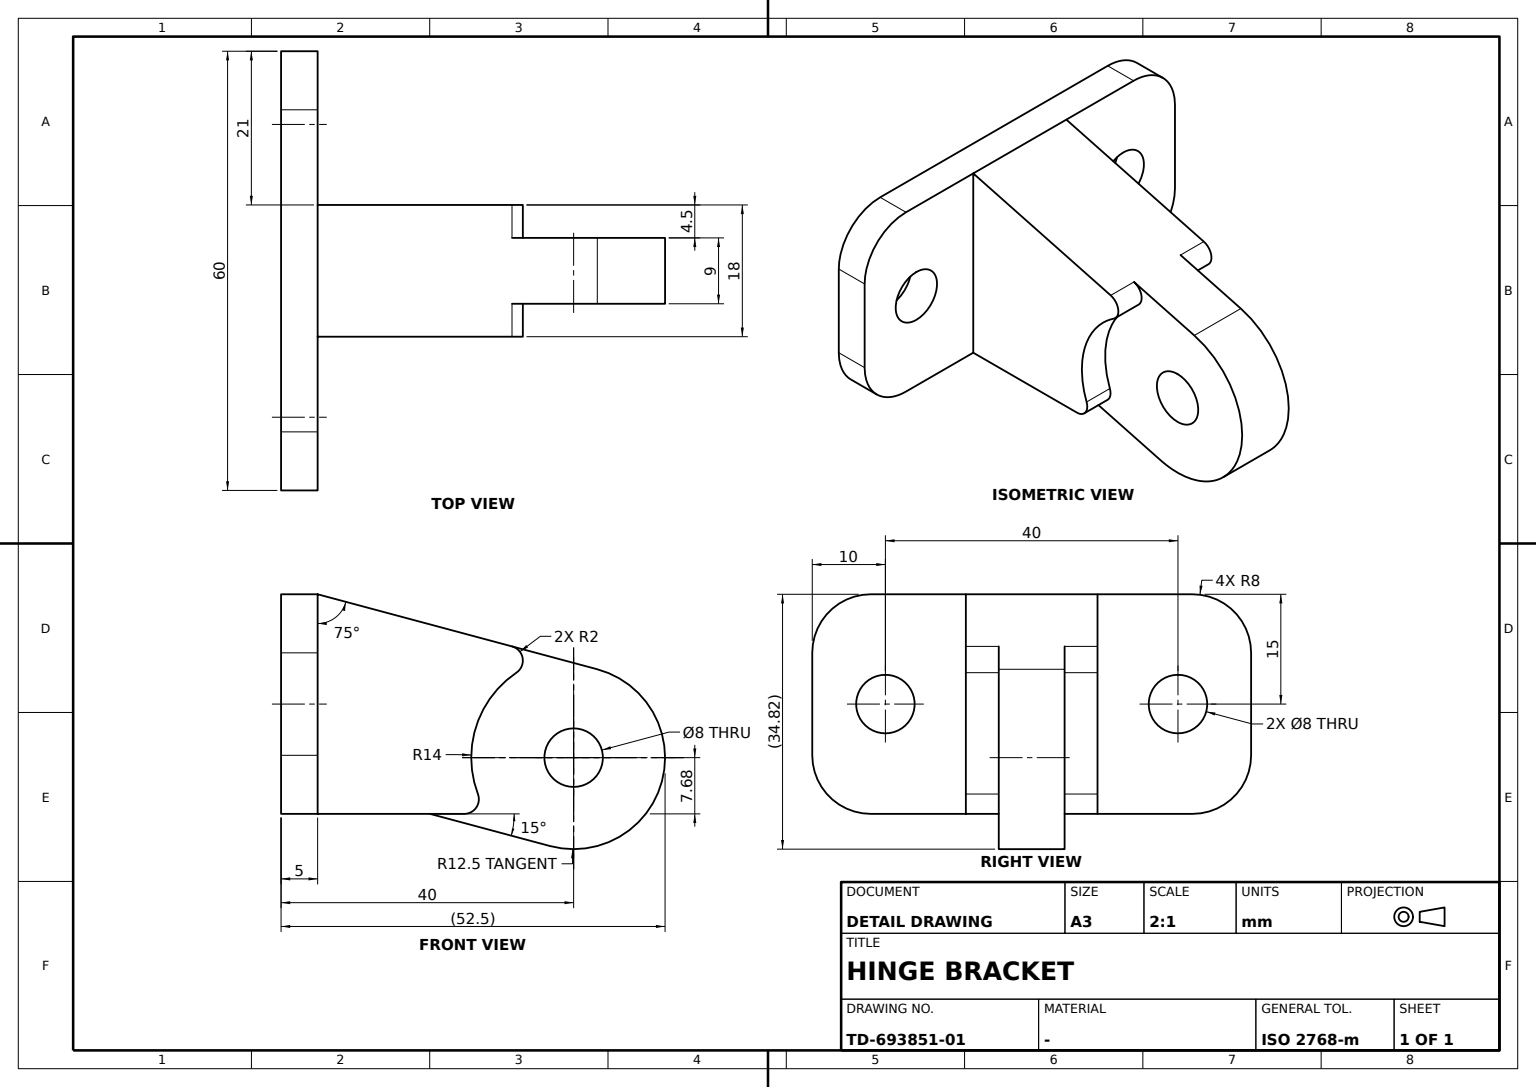
ISO-10303-21;
HEADER;
FILE_DESCRIPTION((''),'2;1');
FILE_NAME('','',(''),(''),'','','');
FILE_SCHEMA(('AUTOMOTIVE_DESIGN'));
ENDSEC;
DATA;
#1=APPLICATION_CONTEXT('');
#2=PRODUCT_CONTEXT('',#1,'mechanical');
#3=PRODUCT('','','',(#2));
#4=PRODUCT_DEFINITION_FORMATION('','',#3);
#5=PRODUCT_DEFINITION_CONTEXT('',#1,'design');
#6=PRODUCT_DEFINITION('','',#4,#5);
#7=PRODUCT_DEFINITION_SHAPE('','',#6);
#8=(LENGTH_UNIT()NAMED_UNIT(*)SI_UNIT(.MILLI.,.METRE.));
#9=(NAMED_UNIT(*)PLANE_ANGLE_UNIT()SI_UNIT($,.RADIAN.));
#10=(NAMED_UNIT(*)SI_UNIT($,.STERADIAN.)SOLID_ANGLE_UNIT());
#11=UNCERTAINTY_MEASURE_WITH_UNIT(LENGTH_MEASURE(0.005),#8,'distance_accuracy_value','');
#12=(GEOMETRIC_REPRESENTATION_CONTEXT(3)GLOBAL_UNCERTAINTY_ASSIGNED_CONTEXT((#11))GLOBAL_UNIT_ASSIGNED_CONTEXT((#8,#9,#10))REPRESENTATION_CONTEXT('',''));
#13=CARTESIAN_POINT('',(-4.5,-25.042453,-15.));
#14=VERTEX_POINT('',#13);
#15=CARTESIAN_POINT('',(-9.,-25.042453,-15.));
#16=VERTEX_POINT('',#15);
#17=CARTESIAN_POINT('',(9.,-25.042453,-15.));
#18=DIRECTION('',(-1.,0.,0.));
#19=VECTOR('',#18,1000.);
#20=LINE('',#17,#19);
#21=EDGE_CURVE('',#14,#16,#20,.T.);
#22=ORIENTED_EDGE('',*,*,#21,.F.);
#23=CARTESIAN_POINT('',(-4.5,-26.912146,-12.289897));
#24=VERTEX_POINT('',#23);
#25=CARTESIAN_POINT('',(-4.5,-25.042453,-13.));
#26=DIRECTION('',(0.,0.,1.));
#27=AXIS2_PLACEMENT_3D('',#25,#18,#26);
#28=CIRCLE('',#27,2.);
#29=EDGE_CURVE('',#14,#24,#28,.T.);
#30=ORIENTED_EDGE('',*,*,#29,.T.);
#31=CARTESIAN_POINT('',(-9.,-26.912146,-12.289897));
#32=VERTEX_POINT('',#31);
#33=CARTESIAN_POINT('',(9.,-26.912146,-12.289897));
#34=LINE('',#33,#19);
#35=EDGE_CURVE('',#24,#32,#34,.T.);
#36=ORIENTED_EDGE('',*,*,#35,.T.);
#37=CARTESIAN_POINT('',(-9.,-25.042453,-13.));
#38=DIRECTION('',(1.,0.,0.));
#39=DIRECTION('',(0.,1.,0.));
#40=AXIS2_PLACEMENT_3D('',#37,#38,#39);
#41=CIRCLE('',#40,2.);
#42=EDGE_CURVE('',#32,#16,#41,.T.);
#43=ORIENTED_EDGE('',*,*,#42,.T.);
#44=EDGE_LOOP('',(#22,#30,#36,#43));
#45=FACE_BOUND('',#44,.T.);
#46=CARTESIAN_POINT('',(9.,-25.042453,-13.));
#47=AXIS2_PLACEMENT_3D('',#46,#18,#26);
#48=CYLINDRICAL_SURFACE('',#47,2.);
#49=ADVANCED_FACE('',(#45),#48,.T.);
#50=CARTESIAN_POINT('',(-20.,-5.,-4.));
#51=VERTEX_POINT('',#50);
#52=CARTESIAN_POINT('',(-20.,-5.,4.));
#53=VERTEX_POINT('',#52);
#54=CARTESIAN_POINT('',(-20.,-5.,0.));
#55=DIRECTION('',(0.,-1.,0.));
#56=AXIS2_PLACEMENT_3D('',#54,#55,#38);
#57=CIRCLE('',#56,4.);
#58=EDGE_CURVE('',#51,#53,#57,.T.);
#59=ORIENTED_EDGE('',*,*,#58,.F.);
#60=EDGE_CURVE('',#53,#51,#57,.T.);
#61=ORIENTED_EDGE('',*,*,#60,.F.);
#62=EDGE_LOOP('',(#59,#61));
#63=FACE_BOUND('',#62,.T.);
#64=CARTESIAN_POINT('',(-9.,-5.,15.));
#65=VERTEX_POINT('',#64);
#66=CARTESIAN_POINT('',(-22.,-5.,15.));
#67=VERTEX_POINT('',#66);
#68=CARTESIAN_POINT('',(22.,-5.,15.));
#69=LINE('',#68,#19);
#70=EDGE_CURVE('',#65,#67,#69,.T.);
#71=ORIENTED_EDGE('',*,*,#70,.T.);
#72=CARTESIAN_POINT('',(-30.,-5.,7.));
#73=VERTEX_POINT('',#72);
#74=CARTESIAN_POINT('',(-22.,-5.,7.));
#75=AXIS2_PLACEMENT_3D('',#74,#55,#38);
#76=CIRCLE('',#75,8.);
#77=EDGE_CURVE('',#67,#73,#76,.T.);
#78=ORIENTED_EDGE('',*,*,#77,.T.);
#79=CARTESIAN_POINT('',(-30.,-5.,-7.));
#80=VERTEX_POINT('',#79);
#81=DIRECTION('',(0.,0.,-1.));
#82=VECTOR('',#81,1000.);
#83=LINE('',#72,#82);
#84=EDGE_CURVE('',#73,#80,#83,.T.);
#85=ORIENTED_EDGE('',*,*,#84,.T.);
#86=CARTESIAN_POINT('',(-22.,-5.,-15.));
#87=VERTEX_POINT('',#86);
#88=CARTESIAN_POINT('',(-22.,-5.,-7.));
#89=AXIS2_PLACEMENT_3D('',#88,#55,#38);
#90=CIRCLE('',#89,8.);
#91=EDGE_CURVE('',#80,#87,#90,.T.);
#92=ORIENTED_EDGE('',*,*,#91,.T.);
#93=CARTESIAN_POINT('',(-9.,-5.,-15.));
#94=VERTEX_POINT('',#93);
#95=VECTOR('',#38,1000.);
#96=LINE('',#86,#95);
#97=EDGE_CURVE('',#87,#94,#96,.T.);
#98=ORIENTED_EDGE('',*,*,#97,.T.);
#99=VECTOR('',#26,1000.);
#100=LINE('',#93,#99);
#101=EDGE_CURVE('',#94,#65,#100,.T.);
#102=ORIENTED_EDGE('',*,*,#101,.T.);
#103=EDGE_LOOP('',(#71,#78,#85,#92,#98,#102));
#104=FACE_BOUND('',#103,.T.);
#105=AXIS2_PLACEMENT_3D('',#88,#55,#81);
#106=PLANE('',#105);
#107=ADVANCED_FACE('',(#63,#104),#106,.T.);
#108=CARTESIAN_POINT('',(-4.5,-40.,-3.319174));
#109=VERTEX_POINT('',#108);
#110=CARTESIAN_POINT('',(-4.5,-40.,-11.319174));
#111=VERTEX_POINT('',#110);
#112=CARTESIAN_POINT('',(-4.5,-40.,-7.319174));
#113=AXIS2_PLACEMENT_3D('',#112,#38,#39);
#114=CIRCLE('',#113,4.);
#115=EDGE_CURVE('',#109,#111,#114,.T.);
#116=ORIENTED_EDGE('',*,*,#115,.F.);
#117=CARTESIAN_POINT('',(4.5,-40.,-3.319174));
#118=VERTEX_POINT('',#117);
#119=LINE('',#117,#19);
#120=EDGE_CURVE('',#118,#109,#119,.T.);
#121=ORIENTED_EDGE('',*,*,#120,.F.);
#122=CARTESIAN_POINT('',(4.5,-40.,-11.319174));
#123=VERTEX_POINT('',#122);
#124=CARTESIAN_POINT('',(4.5,-40.,-7.319174));
#125=AXIS2_PLACEMENT_3D('',#124,#38,#39);
#126=CIRCLE('',#125,4.);
#127=EDGE_CURVE('',#118,#123,#126,.T.);
#128=ORIENTED_EDGE('',*,*,#127,.T.);
#129=LINE('',#122,#19);
#130=EDGE_CURVE('',#111,#123,#129,.F.);
#131=ORIENTED_EDGE('',*,*,#130,.F.);
#132=EDGE_LOOP('',(#116,#121,#128,#131));
#133=FACE_BOUND('',#132,.T.);
#134=AXIS2_PLACEMENT_3D('',#124,#18,#26);
#135=CYLINDRICAL_SURFACE('',#134,4.);
#136=ADVANCED_FACE('',(#133),#135,.F.);
#137=CARTESIAN_POINT('',(-30.,0.,-7.));
#138=VERTEX_POINT('',#137);
#139=VECTOR('',#55,1000.);
#140=LINE('',#137,#139);
#141=EDGE_CURVE('',#138,#80,#140,.T.);
#142=ORIENTED_EDGE('',*,*,#141,.F.);
#143=CARTESIAN_POINT('',(-22.,0.,-15.));
#144=VERTEX_POINT('',#143);
#145=CARTESIAN_POINT('',(-22.,0.,-7.));
#146=AXIS2_PLACEMENT_3D('',#145,#55,#38);
#147=CIRCLE('',#146,8.);
#148=EDGE_CURVE('',#138,#144,#147,.T.);
#149=ORIENTED_EDGE('',*,*,#148,.T.);
#150=LINE('',#143,#139);
#151=EDGE_CURVE('',#144,#87,#150,.T.);
#152=ORIENTED_EDGE('',*,*,#151,.T.);
#153=ORIENTED_EDGE('',*,*,#91,.F.);
#154=EDGE_LOOP('',(#142,#149,#152,#153));
#155=FACE_BOUND('',#154,.T.);
#156=AXIS2_PLACEMENT_3D('',#145,#55,#81);
#157=CYLINDRICAL_SURFACE('',#156,8.);
#158=ADVANCED_FACE('',(#155),#157,.T.);
#159=CARTESIAN_POINT('',(22.,0.,-15.));
#160=VERTEX_POINT('',#159);
#161=LINE('',#143,#95);
#162=EDGE_CURVE('',#144,#160,#161,.T.);
#163=ORIENTED_EDGE('',*,*,#162,.T.);
#164=CARTESIAN_POINT('',(22.,-5.,-15.));
#165=VERTEX_POINT('',#164);
#166=LINE('',#159,#139);
#167=EDGE_CURVE('',#160,#165,#166,.T.);
#168=ORIENTED_EDGE('',*,*,#167,.T.);
#169=CARTESIAN_POINT('',(9.,-5.,-15.));
#170=VERTEX_POINT('',#169);
#171=EDGE_CURVE('',#170,#165,#96,.T.);
#172=ORIENTED_EDGE('',*,*,#171,.F.);
#173=VERTEX_POINT('',#17);
#174=VECTOR('',#39,1000.);
#175=LINE('',#17,#174);
#176=EDGE_CURVE('',#173,#170,#175,.T.);
#177=ORIENTED_EDGE('',*,*,#176,.F.);
#178=CARTESIAN_POINT('',(4.5,-25.042453,-15.));
#179=VERTEX_POINT('',#178);
#180=EDGE_CURVE('',#173,#179,#20,.T.);
#181=ORIENTED_EDGE('',*,*,#180,.T.);
#182=CARTESIAN_POINT('',(4.5,-20.368942,-15.));
#183=VERTEX_POINT('',#182);
#184=LINE('',#182,#139);
#185=EDGE_CURVE('',#183,#179,#184,.T.);
#186=ORIENTED_EDGE('',*,*,#185,.F.);
#187=CARTESIAN_POINT('',(-4.5,-20.368942,-15.));
#188=VERTEX_POINT('',#187);
#189=LINE('',#182,#19);
#190=EDGE_CURVE('',#183,#188,#189,.T.);
#191=ORIENTED_EDGE('',*,*,#190,.T.);
#192=LINE('',#187,#139);
#193=EDGE_CURVE('',#188,#14,#192,.T.);
#194=ORIENTED_EDGE('',*,*,#193,.T.);
#195=ORIENTED_EDGE('',*,*,#21,.T.);
#196=LINE('',#15,#174);
#197=EDGE_CURVE('',#16,#94,#196,.T.);
#198=ORIENTED_EDGE('',*,*,#197,.T.);
#199=ORIENTED_EDGE('',*,*,#97,.F.);
#200=ORIENTED_EDGE('',*,*,#151,.F.);
#201=EDGE_LOOP('',(#163,#168,#172,#177,#181,#186,#191,#194,#195,#198,#199,#200));
#202=FACE_BOUND('',#201,.T.);
#203=AXIS2_PLACEMENT_3D('',#143,#81,#18);
#204=PLANE('',#203);
#205=ADVANCED_FACE('',(#202),#204,.T.);
#206=ORIENTED_EDGE('',*,*,#77,.F.);
#207=CARTESIAN_POINT('',(-22.,0.,15.));
#208=VERTEX_POINT('',#207);
#209=LINE('',#207,#139);
#210=EDGE_CURVE('',#208,#67,#209,.T.);
#211=ORIENTED_EDGE('',*,*,#210,.F.);
#212=CARTESIAN_POINT('',(-30.,0.,7.));
#213=VERTEX_POINT('',#212);
#214=CARTESIAN_POINT('',(-22.,0.,7.));
#215=AXIS2_PLACEMENT_3D('',#214,#55,#38);
#216=CIRCLE('',#215,8.);
#217=EDGE_CURVE('',#208,#213,#216,.T.);
#218=ORIENTED_EDGE('',*,*,#217,.T.);
#219=LINE('',#212,#139);
#220=EDGE_CURVE('',#213,#73,#219,.T.);
#221=ORIENTED_EDGE('',*,*,#220,.T.);
#222=EDGE_LOOP('',(#206,#211,#218,#221));
#223=FACE_BOUND('',#222,.T.);
#224=AXIS2_PLACEMENT_3D('',#214,#55,#81);
#225=CYLINDRICAL_SURFACE('',#224,8.);
#226=ADVANCED_FACE('',(#223),#225,.T.);
#227=ORIENTED_EDGE('',*,*,#180,.F.);
#228=VERTEX_POINT('',#33);
#229=AXIS2_PLACEMENT_3D('',#46,#38,#39);
#230=CIRCLE('',#229,2.);
#231=EDGE_CURVE('',#228,#173,#230,.T.);
#232=ORIENTED_EDGE('',*,*,#231,.F.);
#233=CARTESIAN_POINT('',(4.5,-26.912146,-12.289897));
#234=VERTEX_POINT('',#233);
#235=EDGE_CURVE('',#228,#234,#34,.T.);
#236=ORIENTED_EDGE('',*,*,#235,.T.);
#237=CARTESIAN_POINT('',(4.5,-25.042453,-13.));
#238=AXIS2_PLACEMENT_3D('',#237,#18,#26);
#239=CIRCLE('',#238,2.);
#240=EDGE_CURVE('',#179,#234,#239,.T.);
#241=ORIENTED_EDGE('',*,*,#240,.F.);
#242=EDGE_LOOP('',(#227,#232,#236,#241));
#243=FACE_BOUND('',#242,.T.);
#244=ADVANCED_FACE('',(#243),#48,.T.);
#245=ORIENTED_EDGE('',*,*,#171,.T.);
#246=CARTESIAN_POINT('',(30.,-5.,-7.));
#247=VERTEX_POINT('',#246);
#248=CARTESIAN_POINT('',(22.,-5.,-7.));
#249=AXIS2_PLACEMENT_3D('',#248,#55,#38);
#250=CIRCLE('',#249,8.);
#251=EDGE_CURVE('',#165,#247,#250,.T.);
#252=ORIENTED_EDGE('',*,*,#251,.T.);
#253=CARTESIAN_POINT('',(30.,-5.,7.));
#254=VERTEX_POINT('',#253);
#255=LINE('',#246,#99);
#256=EDGE_CURVE('',#247,#254,#255,.T.);
#257=ORIENTED_EDGE('',*,*,#256,.T.);
#258=VERTEX_POINT('',#68);
#259=CARTESIAN_POINT('',(22.,-5.,7.));
#260=AXIS2_PLACEMENT_3D('',#259,#55,#38);
#261=CIRCLE('',#260,8.);
#262=EDGE_CURVE('',#254,#258,#261,.T.);
#263=ORIENTED_EDGE('',*,*,#262,.T.);
#264=CARTESIAN_POINT('',(9.,-5.,15.));
#265=VERTEX_POINT('',#264);
#266=EDGE_CURVE('',#258,#265,#69,.T.);
#267=ORIENTED_EDGE('',*,*,#266,.T.);
#268=LINE('',#169,#99);
#269=EDGE_CURVE('',#170,#265,#268,.T.);
#270=ORIENTED_EDGE('',*,*,#269,.F.);
#271=EDGE_LOOP('',(#245,#252,#257,#263,#267,#270));
#272=FACE_BOUND('',#271,.T.);
#273=CARTESIAN_POINT('',(20.,-5.,-4.));
#274=VERTEX_POINT('',#273);
#275=CARTESIAN_POINT('',(20.,-5.,4.));
#276=VERTEX_POINT('',#275);
#277=CARTESIAN_POINT('',(20.,-5.,0.));
#278=AXIS2_PLACEMENT_3D('',#277,#55,#38);
#279=CIRCLE('',#278,4.);
#280=EDGE_CURVE('',#274,#276,#279,.T.);
#281=ORIENTED_EDGE('',*,*,#280,.F.);
#282=EDGE_CURVE('',#276,#274,#279,.T.);
#283=ORIENTED_EDGE('',*,*,#282,.F.);
#284=EDGE_LOOP('',(#281,#283));
#285=FACE_BOUND('',#284,.T.);
#286=ADVANCED_FACE('',(#272,#285),#106,.T.);
#287=ORIENTED_EDGE('',*,*,#185,.T.);
#288=ORIENTED_EDGE('',*,*,#240,.T.);
#289=CARTESIAN_POINT('',(4.5,-32.174237,4.289333));
#290=VERTEX_POINT('',#289);
#291=AXIS2_PLACEMENT_3D('',#124,#38,#26);
#292=CIRCLE('',#291,14.);
#293=EDGE_CURVE('',#234,#290,#292,.T.);
#294=ORIENTED_EDGE('',*,*,#293,.T.);
#295=CARTESIAN_POINT('',(4.5,-31.573909,7.879543));
#296=VERTEX_POINT('',#295);
#297=CARTESIAN_POINT('',(4.5,-31.056271,5.947691));
#298=AXIS2_PLACEMENT_3D('',#297,#18,#26);
#299=CIRCLE('',#298,2.);
#300=EDGE_CURVE('',#290,#296,#299,.T.);
#301=ORIENTED_EDGE('',*,*,#300,.T.);
#302=CARTESIAN_POINT('',(4.5,-43.235238,4.754899));
#303=VERTEX_POINT('',#302);
#304=DIRECTION('',(0.,-0.965925826,-0.258819045));
#305=VECTOR('',#304,1000.);
#306=LINE('',#295,#305);
#307=EDGE_CURVE('',#296,#303,#306,.T.);
#308=ORIENTED_EDGE('',*,*,#307,.T.);
#309=CARTESIAN_POINT('',(4.5,-36.764762,-19.393247));
#310=VERTEX_POINT('',#309);
#311=CIRCLE('',#125,12.5);
#312=EDGE_CURVE('',#303,#310,#311,.T.);
#313=ORIENTED_EDGE('',*,*,#312,.T.);
#314=DIRECTION('',(0.,0.965925826,0.258819045));
#315=VECTOR('',#314,1000.);
#316=LINE('',#309,#315);
#317=EDGE_CURVE('',#310,#183,#316,.T.);
#318=ORIENTED_EDGE('',*,*,#317,.T.);
#319=EDGE_LOOP('',(#287,#288,#294,#301,#308,#313,#318));
#320=FACE_BOUND('',#319,.T.);
#321=EDGE_CURVE('',#123,#118,#126,.T.);
#322=ORIENTED_EDGE('',*,*,#321,.F.);
#323=ORIENTED_EDGE('',*,*,#127,.F.);
#324=EDGE_LOOP('',(#322,#323));
#325=FACE_BOUND('',#324,.T.);
#326=AXIS2_PLACEMENT_3D('',#124,#38,#81);
#327=PLANE('',#326);
#328=ADVANCED_FACE('',(#320,#325),#327,.T.);
#329=CARTESIAN_POINT('',(-20.,0.,4.));
#330=VERTEX_POINT('',#329);
#331=CARTESIAN_POINT('',(-20.,0.,-4.));
#332=VERTEX_POINT('',#331);
#333=CARTESIAN_POINT('',(-20.,0.,0.));
#334=AXIS2_PLACEMENT_3D('',#333,#55,#38);
#335=CIRCLE('',#334,4.);
#336=EDGE_CURVE('',#330,#332,#335,.T.);
#337=ORIENTED_EDGE('',*,*,#336,.F.);
#338=LINE('',#329,#139);
#339=EDGE_CURVE('',#330,#53,#338,.T.);
#340=ORIENTED_EDGE('',*,*,#339,.T.);
#341=ORIENTED_EDGE('',*,*,#60,.T.);
#342=LINE('',#331,#139);
#343=EDGE_CURVE('',#51,#332,#342,.F.);
#344=ORIENTED_EDGE('',*,*,#343,.T.);
#345=EDGE_LOOP('',(#337,#340,#341,#344));
#346=FACE_BOUND('',#345,.T.);
#347=AXIS2_PLACEMENT_3D('',#333,#55,#81);
#348=CYLINDRICAL_SURFACE('',#347,4.);
#349=ADVANCED_FACE('',(#346),#348,.F.);
#350=CARTESIAN_POINT('',(-4.5,-32.174237,4.289333));
#351=VERTEX_POINT('',#350);
#352=CARTESIAN_POINT('',(-9.,-32.174237,4.289333));
#353=VERTEX_POINT('',#352);
#354=CARTESIAN_POINT('',(9.,-32.174237,4.289333));
#355=LINE('',#354,#19);
#356=EDGE_CURVE('',#351,#353,#355,.T.);
#357=ORIENTED_EDGE('',*,*,#356,.T.);
#358=CARTESIAN_POINT('',(-9.,-40.,-7.319174));
#359=AXIS2_PLACEMENT_3D('',#358,#18,#39);
#360=CIRCLE('',#359,14.);
#361=EDGE_CURVE('',#353,#32,#360,.T.);
#362=ORIENTED_EDGE('',*,*,#361,.T.);
#363=ORIENTED_EDGE('',*,*,#35,.F.);
#364=AXIS2_PLACEMENT_3D('',#112,#38,#26);
#365=CIRCLE('',#364,14.);
#366=EDGE_CURVE('',#24,#351,#365,.T.);
#367=ORIENTED_EDGE('',*,*,#366,.T.);
#368=EDGE_LOOP('',(#357,#362,#363,#367));
#369=FACE_BOUND('',#368,.T.);
#370=CARTESIAN_POINT('',(9.,-40.,-7.319174));
#371=AXIS2_PLACEMENT_3D('',#370,#18,#26);
#372=CYLINDRICAL_SURFACE('',#371,14.);
#373=ADVANCED_FACE('',(#369),#372,.F.);
#374=ORIENTED_EDGE('',*,*,#321,.T.);
#375=ORIENTED_EDGE('',*,*,#120,.T.);
#376=EDGE_CURVE('',#111,#109,#114,.T.);
#377=ORIENTED_EDGE('',*,*,#376,.F.);
#378=ORIENTED_EDGE('',*,*,#130,.T.);
#379=EDGE_LOOP('',(#374,#375,#377,#378));
#380=FACE_BOUND('',#379,.T.);
#381=ADVANCED_FACE('',(#380),#135,.F.);
#382=ORIENTED_EDGE('',*,*,#101,.F.);
#383=ORIENTED_EDGE('',*,*,#197,.F.);
#384=ORIENTED_EDGE('',*,*,#42,.F.);
#385=ORIENTED_EDGE('',*,*,#361,.F.);
#386=CARTESIAN_POINT('',(-9.,-31.573909,7.879543));
#387=VERTEX_POINT('',#386);
#388=CARTESIAN_POINT('',(-9.,-31.056271,5.947691));
#389=AXIS2_PLACEMENT_3D('',#388,#38,#39);
#390=CIRCLE('',#389,2.);
#391=EDGE_CURVE('',#387,#353,#390,.T.);
#392=ORIENTED_EDGE('',*,*,#391,.F.);
#393=LINE('',#64,#305);
#394=EDGE_CURVE('',#65,#387,#393,.T.);
#395=ORIENTED_EDGE('',*,*,#394,.F.);
#396=EDGE_LOOP('',(#382,#383,#384,#385,#392,#395));
#397=FACE_BOUND('',#396,.T.);
#398=AXIS2_PLACEMENT_3D('',#388,#38,#81);
#399=PLANE('',#398);
#400=ADVANCED_FACE('',(#397),#399,.F.);
#401=ORIENTED_EDGE('',*,*,#293,.F.);
#402=ORIENTED_EDGE('',*,*,#235,.F.);
#403=VERTEX_POINT('',#354);
#404=AXIS2_PLACEMENT_3D('',#370,#18,#39);
#405=CIRCLE('',#404,14.);
#406=EDGE_CURVE('',#403,#228,#405,.T.);
#407=ORIENTED_EDGE('',*,*,#406,.F.);
#408=EDGE_CURVE('',#403,#290,#355,.T.);
#409=ORIENTED_EDGE('',*,*,#408,.T.);
#410=EDGE_LOOP('',(#401,#402,#407,#409));
#411=FACE_BOUND('',#410,.T.);
#412=ADVANCED_FACE('',(#411),#372,.F.);
#413=ORIENTED_EDGE('',*,*,#190,.F.);
#414=ORIENTED_EDGE('',*,*,#317,.F.);
#415=CARTESIAN_POINT('',(-4.5,-36.764762,-19.393247));
#416=VERTEX_POINT('',#415);
#417=LINE('',#309,#19);
#418=EDGE_CURVE('',#310,#416,#417,.T.);
#419=ORIENTED_EDGE('',*,*,#418,.T.);
#420=LINE('',#415,#315);
#421=EDGE_CURVE('',#416,#188,#420,.T.);
#422=ORIENTED_EDGE('',*,*,#421,.T.);
#423=EDGE_LOOP('',(#413,#414,#419,#422));
#424=FACE_BOUND('',#423,.T.);
#425=DIRECTION('',(0.,-0.258819045,0.965925826));
#426=AXIS2_PLACEMENT_3D('',#309,#425,#304);
#427=PLANE('',#426);
#428=ADVANCED_FACE('',(#424),#427,.F.);
#429=CARTESIAN_POINT('',(20.,0.,4.));
#430=VERTEX_POINT('',#429);
#431=LINE('',#429,#139);
#432=EDGE_CURVE('',#276,#430,#431,.F.);
#433=ORIENTED_EDGE('',*,*,#432,.T.);
#434=CARTESIAN_POINT('',(20.,0.,-4.));
#435=VERTEX_POINT('',#434);
#436=CARTESIAN_POINT('',(20.,0.,0.));
#437=AXIS2_PLACEMENT_3D('',#436,#55,#38);
#438=CIRCLE('',#437,4.);
#439=EDGE_CURVE('',#435,#430,#438,.T.);
#440=ORIENTED_EDGE('',*,*,#439,.F.);
#441=LINE('',#434,#139);
#442=EDGE_CURVE('',#435,#274,#441,.T.);
#443=ORIENTED_EDGE('',*,*,#442,.T.);
#444=ORIENTED_EDGE('',*,*,#280,.T.);
#445=EDGE_LOOP('',(#433,#440,#443,#444));
#446=FACE_BOUND('',#445,.T.);
#447=AXIS2_PLACEMENT_3D('',#436,#55,#81);
#448=CYLINDRICAL_SURFACE('',#447,4.);
#449=ADVANCED_FACE('',(#446),#448,.F.);
#450=CARTESIAN_POINT('',(22.,0.,15.));
#451=VERTEX_POINT('',#450);
#452=LINE('',#450,#139);
#453=EDGE_CURVE('',#451,#258,#452,.T.);
#454=ORIENTED_EDGE('',*,*,#453,.F.);
#455=LINE('',#450,#19);
#456=EDGE_CURVE('',#451,#208,#455,.T.);
#457=ORIENTED_EDGE('',*,*,#456,.T.);
#458=ORIENTED_EDGE('',*,*,#210,.T.);
#459=ORIENTED_EDGE('',*,*,#70,.F.);
#460=LINE('',#264,#19);
#461=EDGE_CURVE('',#265,#65,#460,.T.);
#462=ORIENTED_EDGE('',*,*,#461,.F.);
#463=ORIENTED_EDGE('',*,*,#266,.F.);
#464=EDGE_LOOP('',(#454,#457,#458,#459,#462,#463));
#465=FACE_BOUND('',#464,.T.);
#466=AXIS2_PLACEMENT_3D('',#450,#26,#38);
#467=PLANE('',#466);
#468=ADVANCED_FACE('',(#465),#467,.T.);
#469=ORIENTED_EDGE('',*,*,#231,.T.);
#470=ORIENTED_EDGE('',*,*,#176,.T.);
#471=ORIENTED_EDGE('',*,*,#269,.T.);
#472=CARTESIAN_POINT('',(9.,-31.573909,7.879543));
#473=VERTEX_POINT('',#472);
#474=LINE('',#264,#305);
#475=EDGE_CURVE('',#265,#473,#474,.T.);
#476=ORIENTED_EDGE('',*,*,#475,.T.);
#477=CARTESIAN_POINT('',(9.,-31.056271,5.947691));
#478=AXIS2_PLACEMENT_3D('',#477,#38,#39);
#479=CIRCLE('',#478,2.);
#480=EDGE_CURVE('',#473,#403,#479,.T.);
#481=ORIENTED_EDGE('',*,*,#480,.T.);
#482=ORIENTED_EDGE('',*,*,#406,.T.);
#483=EDGE_LOOP('',(#469,#470,#471,#476,#481,#482));
#484=FACE_BOUND('',#483,.T.);
#485=AXIS2_PLACEMENT_3D('',#477,#38,#81);
#486=PLANE('',#485);
#487=ADVANCED_FACE('',(#484),#486,.T.);
#488=ORIENTED_EDGE('',*,*,#84,.F.);
#489=ORIENTED_EDGE('',*,*,#220,.F.);
#490=LINE('',#212,#82);
#491=EDGE_CURVE('',#213,#138,#490,.T.);
#492=ORIENTED_EDGE('',*,*,#491,.T.);
#493=ORIENTED_EDGE('',*,*,#141,.T.);
#494=EDGE_LOOP('',(#488,#489,#492,#493));
#495=FACE_BOUND('',#494,.T.);
#496=AXIS2_PLACEMENT_3D('',#212,#18,#26);
#497=PLANE('',#496);
#498=ADVANCED_FACE('',(#495),#497,.T.);
#499=ORIENTED_EDGE('',*,*,#439,.T.);
#500=EDGE_CURVE('',#430,#435,#438,.T.);
#501=ORIENTED_EDGE('',*,*,#500,.T.);
#502=EDGE_LOOP('',(#499,#501));
#503=FACE_BOUND('',#502,.T.);
#504=ORIENTED_EDGE('',*,*,#148,.F.);
#505=ORIENTED_EDGE('',*,*,#491,.F.);
#506=ORIENTED_EDGE('',*,*,#217,.F.);
#507=ORIENTED_EDGE('',*,*,#456,.F.);
#508=CARTESIAN_POINT('',(30.,0.,7.));
#509=VERTEX_POINT('',#508);
#510=CARTESIAN_POINT('',(22.,0.,7.));
#511=AXIS2_PLACEMENT_3D('',#510,#55,#38);
#512=CIRCLE('',#511,8.);
#513=EDGE_CURVE('',#509,#451,#512,.T.);
#514=ORIENTED_EDGE('',*,*,#513,.F.);
#515=CARTESIAN_POINT('',(30.,0.,-7.));
#516=VERTEX_POINT('',#515);
#517=LINE('',#515,#99);
#518=EDGE_CURVE('',#516,#509,#517,.T.);
#519=ORIENTED_EDGE('',*,*,#518,.F.);
#520=CARTESIAN_POINT('',(22.,0.,-7.));
#521=AXIS2_PLACEMENT_3D('',#520,#55,#38);
#522=CIRCLE('',#521,8.);
#523=EDGE_CURVE('',#160,#516,#522,.T.);
#524=ORIENTED_EDGE('',*,*,#523,.F.);
#525=ORIENTED_EDGE('',*,*,#162,.F.);
#526=EDGE_LOOP('',(#504,#505,#506,#507,#514,#519,#524,#525));
#527=FACE_BOUND('',#526,.T.);
#528=EDGE_CURVE('',#332,#330,#335,.T.);
#529=ORIENTED_EDGE('',*,*,#528,.T.);
#530=ORIENTED_EDGE('',*,*,#336,.T.);
#531=EDGE_LOOP('',(#529,#530));
#532=FACE_BOUND('',#531,.T.);
#533=PLANE('',#156);
#534=ADVANCED_FACE('',(#503,#527,#532),#533,.F.);
#535=LINE('',#472,#19);
#536=EDGE_CURVE('',#473,#296,#535,.T.);
#537=ORIENTED_EDGE('',*,*,#536,.T.);
#538=ORIENTED_EDGE('',*,*,#300,.F.);
#539=ORIENTED_EDGE('',*,*,#408,.F.);
#540=ORIENTED_EDGE('',*,*,#480,.F.);
#541=EDGE_LOOP('',(#537,#538,#539,#540));
#542=FACE_BOUND('',#541,.T.);
#543=AXIS2_PLACEMENT_3D('',#477,#18,#26);
#544=CYLINDRICAL_SURFACE('',#543,2.);
#545=ADVANCED_FACE('',(#542),#544,.T.);
#546=ORIENTED_EDGE('',*,*,#343,.F.);
#547=ORIENTED_EDGE('',*,*,#58,.T.);
#548=ORIENTED_EDGE('',*,*,#339,.F.);
#549=ORIENTED_EDGE('',*,*,#528,.F.);
#550=EDGE_LOOP('',(#546,#547,#548,#549));
#551=FACE_BOUND('',#550,.T.);
#552=ADVANCED_FACE('',(#551),#348,.F.);
#553=ORIENTED_EDGE('',*,*,#432,.F.);
#554=ORIENTED_EDGE('',*,*,#282,.T.);
#555=ORIENTED_EDGE('',*,*,#442,.F.);
#556=ORIENTED_EDGE('',*,*,#500,.F.);
#557=EDGE_LOOP('',(#553,#554,#555,#556));
#558=FACE_BOUND('',#557,.T.);
#559=ADVANCED_FACE('',(#558),#448,.F.);
#560=ORIENTED_EDGE('',*,*,#29,.F.);
#561=ORIENTED_EDGE('',*,*,#193,.F.);
#562=ORIENTED_EDGE('',*,*,#421,.F.);
#563=CARTESIAN_POINT('',(-4.5,-43.235238,4.754899));
#564=VERTEX_POINT('',#563);
#565=CIRCLE('',#113,12.5);
#566=EDGE_CURVE('',#564,#416,#565,.T.);
#567=ORIENTED_EDGE('',*,*,#566,.F.);
#568=CARTESIAN_POINT('',(-4.5,-31.573909,7.879543));
#569=VERTEX_POINT('',#568);
#570=LINE('',#568,#305);
#571=EDGE_CURVE('',#569,#564,#570,.T.);
#572=ORIENTED_EDGE('',*,*,#571,.F.);
#573=CARTESIAN_POINT('',(-4.5,-31.056271,5.947691));
#574=AXIS2_PLACEMENT_3D('',#573,#18,#26);
#575=CIRCLE('',#574,2.);
#576=EDGE_CURVE('',#351,#569,#575,.T.);
#577=ORIENTED_EDGE('',*,*,#576,.F.);
#578=ORIENTED_EDGE('',*,*,#366,.F.);
#579=EDGE_LOOP('',(#560,#561,#562,#567,#572,#577,#578));
#580=FACE_BOUND('',#579,.T.);
#581=ORIENTED_EDGE('',*,*,#115,.T.);
#582=ORIENTED_EDGE('',*,*,#376,.T.);
#583=EDGE_LOOP('',(#581,#582));
#584=FACE_BOUND('',#583,.T.);
#585=AXIS2_PLACEMENT_3D('',#112,#38,#81);
#586=PLANE('',#585);
#587=ADVANCED_FACE('',(#580,#584),#586,.F.);
#588=ORIENTED_EDGE('',*,*,#256,.F.);
#589=LINE('',#515,#139);
#590=EDGE_CURVE('',#516,#247,#589,.T.);
#591=ORIENTED_EDGE('',*,*,#590,.F.);
#592=ORIENTED_EDGE('',*,*,#518,.T.);
#593=LINE('',#508,#139);
#594=EDGE_CURVE('',#509,#254,#593,.T.);
#595=ORIENTED_EDGE('',*,*,#594,.T.);
#596=EDGE_LOOP('',(#588,#591,#592,#595));
#597=FACE_BOUND('',#596,.T.);
#598=AXIS2_PLACEMENT_3D('',#515,#38,#81);
#599=PLANE('',#598);
#600=ADVANCED_FACE('',(#597),#599,.T.);
#601=LINE('',#302,#19);
#602=EDGE_CURVE('',#303,#564,#601,.T.);
#603=ORIENTED_EDGE('',*,*,#602,.T.);
#604=ORIENTED_EDGE('',*,*,#566,.T.);
#605=ORIENTED_EDGE('',*,*,#418,.F.);
#606=ORIENTED_EDGE('',*,*,#312,.F.);
#607=EDGE_LOOP('',(#603,#604,#605,#606));
#608=FACE_BOUND('',#607,.T.);
#609=CYLINDRICAL_SURFACE('',#134,12.5);
#610=ADVANCED_FACE('',(#608),#609,.T.);
#611=ORIENTED_EDGE('',*,*,#513,.T.);
#612=ORIENTED_EDGE('',*,*,#453,.T.);
#613=ORIENTED_EDGE('',*,*,#262,.F.);
#614=ORIENTED_EDGE('',*,*,#594,.F.);
#615=EDGE_LOOP('',(#611,#612,#613,#614));
#616=FACE_BOUND('',#615,.T.);
#617=AXIS2_PLACEMENT_3D('',#510,#55,#81);
#618=CYLINDRICAL_SURFACE('',#617,8.);
#619=ADVANCED_FACE('',(#616),#618,.T.);
#620=ORIENTED_EDGE('',*,*,#167,.F.);
#621=ORIENTED_EDGE('',*,*,#523,.T.);
#622=ORIENTED_EDGE('',*,*,#590,.T.);
#623=ORIENTED_EDGE('',*,*,#251,.F.);
#624=EDGE_LOOP('',(#620,#621,#622,#623));
#625=FACE_BOUND('',#624,.T.);
#626=AXIS2_PLACEMENT_3D('',#520,#55,#81);
#627=CYLINDRICAL_SURFACE('',#626,8.);
#628=ADVANCED_FACE('',(#625),#627,.T.);
#629=EDGE_CURVE('',#569,#387,#535,.T.);
#630=ORIENTED_EDGE('',*,*,#629,.T.);
#631=ORIENTED_EDGE('',*,*,#391,.T.);
#632=ORIENTED_EDGE('',*,*,#356,.F.);
#633=ORIENTED_EDGE('',*,*,#576,.T.);
#634=EDGE_LOOP('',(#630,#631,#632,#633));
#635=FACE_BOUND('',#634,.T.);
#636=ADVANCED_FACE('',(#635),#544,.T.);
#637=ORIENTED_EDGE('',*,*,#536,.F.);
#638=ORIENTED_EDGE('',*,*,#475,.F.);
#639=ORIENTED_EDGE('',*,*,#461,.T.);
#640=ORIENTED_EDGE('',*,*,#394,.T.);
#641=ORIENTED_EDGE('',*,*,#629,.F.);
#642=ORIENTED_EDGE('',*,*,#571,.T.);
#643=ORIENTED_EDGE('',*,*,#602,.F.);
#644=ORIENTED_EDGE('',*,*,#307,.F.);
#645=EDGE_LOOP('',(#637,#638,#639,#640,#641,#642,#643,#644));
#646=FACE_BOUND('',#645,.T.);
#647=DIRECTION('',(0.,0.258819045,-0.965925826));
#648=AXIS2_PLACEMENT_3D('',#264,#647,#314);
#649=PLANE('',#648);
#650=ADVANCED_FACE('',(#646),#649,.F.);
#651=CLOSED_SHELL('',(#49,#107,#136,#158,#205,#226,#244,#286,#328,#349,#373,#381,#400,#412,#428,#449,#468,#487,#498,#534,#545,#552,#559,#587,#600,#610,#619,#628,#636,#650));
#652=MANIFOLD_SOLID_BREP('',#651);
#653=ADVANCED_BREP_SHAPE_REPRESENTATION('',(#652),#12);
#654=SHAPE_DEFINITION_REPRESENTATION(#7,#653);
ENDSEC;
END-ISO-10303-21;
